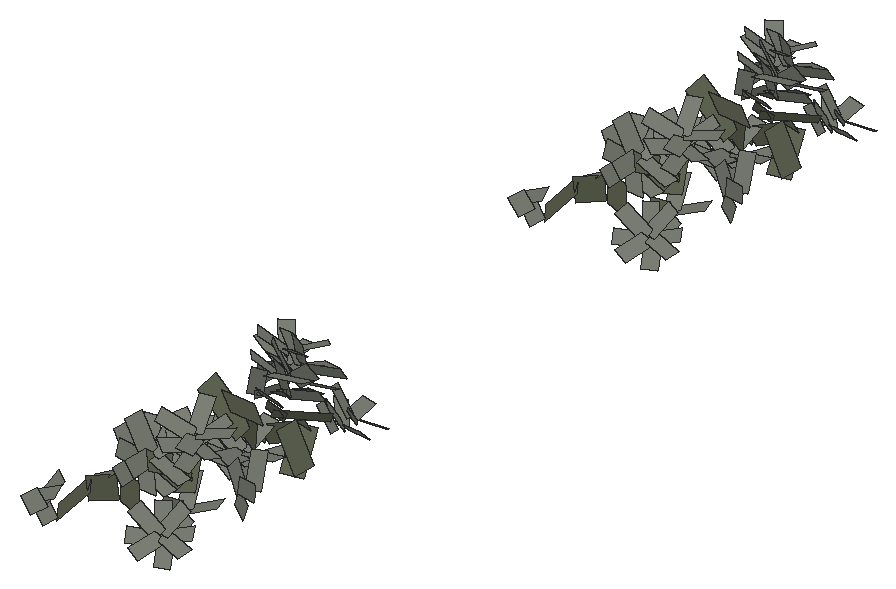
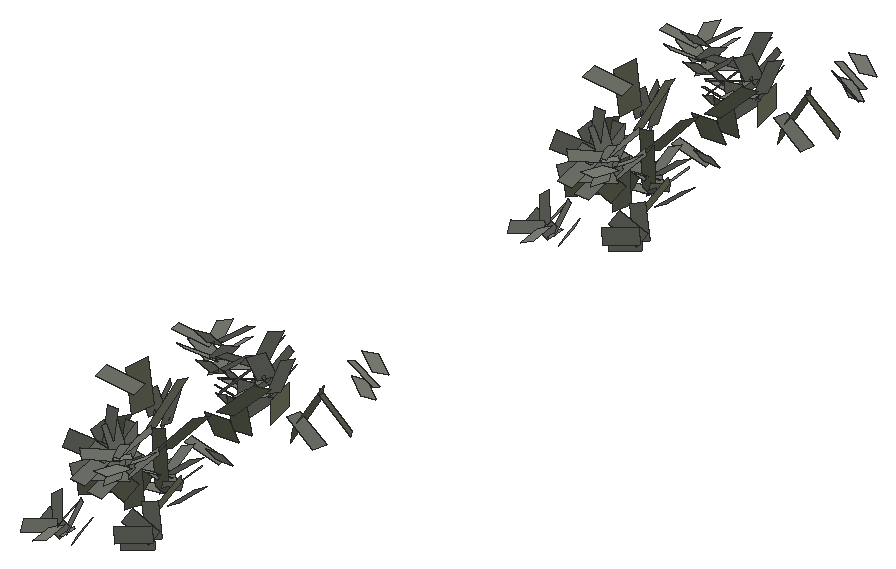
# SketchUp Ruby script. Lengths in inches.
U = 1.inch
M = Sketchup.active_model
def pt(a) = Geom::Point3d.new(a.map { |v| v * U })
def face(e, loops, mat)
  f = e.add_face(loops[0].map { |a| pt(a) })
  loops[1..].each { |l| e.add_face(l.map { |a| pt(a) }).erase! }
  f.material = f.back_material = mat if mat
  f
end
# faces: each face lists its corners as indices into pts; further lists are holes
def faces(e, pts, list, mat = nil) = list.each { |f| face(e, (f[0].is_a?(Array) ? f : [f]).map { |l| l.map { |i| pts[i] } }, mat) }
# xy, xz, yz: faces in a plane at the given z, y or x. An outline is a flat list of corners, or four numbers for a rectangle; further outlines are holes
def ring(l) = l.size == 4 ? [[l[0], l[1]], [l[2], l[1]], [l[2], l[3]], [l[0], l[3]]] : l.each_slice(2).to_a
def flat(e, list, mat, &to3) = list.each { |f| face(e, (f[0].is_a?(Array) ? f : [f]).map { |l| ring(l).map { |u, v| to3.(u, v) } }, mat) }
def xy(e, z, list, mat = nil) = flat(e, list, mat) { |x, y| [x, y, z] }
def xz(e, y, list, mat = nil) = flat(e, list, mat) { |x, z| [x, y, z] }
def yz(e, x, list, mat = nil) = flat(e, list, mat) { |y, z| [x, y, z] }
def lines(e, pts, list) = list.each { |a, b| e.add_line(pt(pts[a]), pt(pts[b])) }
# prism: a flat outline (further loops are holes) pulled along v
def prism(e, loops, v, mat = nil)
  f = face(e, loops, mat); d = Geom::Vector3d.new(v.map { |x| x * U })
  f.pushpull(f.normal.samedirection?(d) ? d.length : -d.length)
end
def box(e, o, s, mat = nil) = prism(e, [[o, [o[0] + s[0], o[1], o[2]], [o[0] + s[0], o[1] + s[1], o[2]], [o[0], o[1] + s[1], o[2]]]], [0, 0, s[2]], mat)
def at(x, y, z, deg = 0) = Geom::Transformation.translation(pt([x, y, z])) * Geom::Transformation.rotation(ORIGIN, Z_AXIS, deg.degrees)
def axes(o, x, y, z) = Geom::Transformation.new([*x, 0, *y, 0, *z, 0, *pt(o).to_a, 1])
def part(name) = M.definitions.add(name)
# library, detail: a bought-in or finely detailed component or shape, given as its bounding box
def library(name, o, s) = part(name).tap { |d| box(d.entities, o, s) }
def detail(e, o, s) = box(e.add_group.entities, o, s)
def put(e, d, t, mat = nil) = e.add_instance(d, t).tap { |i| i.material = mat if mat }
def group(e, t, mat = nil) = e.add_group.tap { |g| g.transformation = t; g.material = mat if mat }.entities
root = M.entities
M.materials.add("viburnumblaasdfas0df1w06d").color = [98, 102, 84]
M.materials.add("viburnumbladsadfasdfad0w122").color = [125, 129, 119]
c1 = part("Component\#315")
p = [[0.25,0,0],[2.05,0.01,0.35],[1.81,4.2,1.66],[0,4.19,1.3125]]
faces(c1.entities,p,[[0,1,2,3]],"viburnumbladsadfasdfad0w122")
c2 = part("viburnumblad2")
put(c2.entities,c1,axes([-19.23,-4.49,-32.18],[83.35428,0,0],[0,79.38502,0],[0,0,83.35428]))
c3 = part("Component\#314")
p = [[0.14,0,0],[2.58,0.05,0.25],[2.44,5.11,2.64],[0,5.05,2.39]]
faces(c3.entities,p,[[0,1,2,3]],"viburnumblaasdfas0df1w06d")
c4 = part("viburnumblad1\#2")
put(c4.entities,c3,axes([-37.25,6.23,19.31],[75.98784,0,0],[0,65.50676,0],[0,0,75.98784]))
put(root,c2,axes([1232.09,187.71,33.1875],[0.01038,-0.0051,-0.00415],[0.00571,0.00633,0.00604],[-0.00053,-0.00802,0.00751]))
put(root,c2,axes([1232.15,299.43,32.05],[0.00525,-0.00588,0.00776],[0.00856,0.00697,-0.00051],[-0.00462,0.00625,0.00786]))
put(root,c2,axes([1232.15,222.55,32.05],[0.00525,-0.00588,0.00776],[0.00856,0.00697,-0.00051],[-0.00462,0.00625,0.00786]))
put(root,c2,axes([1232.11,273.91,31.72],[-0.00042,-0.01207,-0.00346],[0.01224,-0.00117,0.00258],[-0.0028,-0.00328,0.0118]))
put(root,c2,axes([1232.11,197.03,31.72],[-0.00042,-0.01207,-0.00346],[0.01224,-0.00117,0.00258],[-0.0028,-0.00328,0.0118]))
put(root,c2,axes([1233.2,298.68,31.16],[-0.0027,-0.00851,0.00652],[0.00882,0.00097,0.00492],[-0.00475,0.00698,0.00714]))
put(root,c2,axes([1233.2,221.8,31.16],[-0.0027,-0.00851,0.00652],[0.00882,0.00097,0.00492],[-0.00475,0.00698,0.00714]))
put(root,c4,axes([1232.09,268.17,30.0625],[0.00746,-0.00961,-0.00443],[0.01187,0.00604,0.00656],[-0.00274,-0.0068,0.00947]))
put(root,c4,axes([1232.09,191.28,30.0625],[0.00746,-0.00961,-0.00443],[0.01187,0.00604,0.00656],[-0.00274,-0.0068,0.00947]))
put(root,c2,axes([1232.46,263.98,34.32],[0.00254,-0.00908,-0.00688],[0.01053,0.00118,0.00207],[-0.00116,-0.00732,0.00806]))
put(root,c2,axes([1232.46,187.1,34.32],[0.00254,-0.00908,-0.00688],[0.01053,0.00118,0.00207],[-0.00116,-0.00732,0.00806]))
put(root,c2,axes([1234.25,297.67,30.84],[-0.00788,-0.0064,0.00067],[0.00477,-0.00497,0.00864],[-0.00511,0.00701,0.00686]))
put(root,c2,axes([1234.25,220.79,30.84],[-0.00788,-0.0064,0.00067],[0.00477,-0.00497,0.00864],[-0.00511,0.00701,0.00686]))
put(root,c2,axes([1233.36,264.65,33.3],[-0.00572,-0.00664,-0.00612],[0.0099,-0.00571,-0.00294],[-0.00165,-0.00728,0.00803]))
put(root,c2,axes([1233.36,187.76,33.3],[-0.00572,-0.00664,-0.00612],[0.0099,-0.00571,-0.00294],[-0.00165,-0.00728,0.00803]))
put(root,c2,axes([1233.42,262.85,35.21],[-0.00636,-0.00796,-0.00575],[0.0099,-0.00571,-0.00294],[-0.00097,-0.00646,0.0087]))
put(root,c2,axes([1233.42,185.97,35.21],[-0.00636,-0.00796,-0.00575],[0.0099,-0.00571,-0.00294],[-0.00097,-0.00646,0.0087]))
put(root,c2,axes([1233.23,297.71,30.22],[0.00548,-0.00614,0.0081],[0.00771,0.00628,-0.00046],[-0.00462,0.00625,0.00786]))
put(root,c2,axes([1233.23,220.82,30.22],[0.00548,-0.00614,0.0081],[0.00771,0.00628,-0.00046],[-0.00462,0.00625,0.00786]))
put(root,c4,axes([1235.59,273.05,30.45],[-0.00612,0.00474,0.0114],[-0.00511,-0.01476,0.0034],[0.01154,-0.00234,0.00716]))
put(root,c4,axes([1235.59,196.17,30.45],[-0.00612,0.00474,0.0114],[-0.00511,-0.01476,0.0034],[0.01154,-0.00234,0.00716]))
put(root,c4,axes([1238.55,292.45,28.96],[-0.00897,0.00933,0.00213],[-0.00926,-0.01033,0.00624],[0.00527,0.00238,0.01177]))
put(root,c4,axes([1238.55,215.5625,28.96],[-0.00897,0.00933,0.00213],[-0.00926,-0.01033,0.00624],[0.00527,0.00238,0.01177]))
put(root,c2,axes([1238.65,294.53,37.13],[0.0001,0.01076,-0.00253],[-0.0107,0.00082,0.00309],[0.00316,0.0024,0.01032]))
put(root,c2,axes([1238.65,217.65,37.13],[0.0001,0.01076,-0.00253],[-0.0107,0.00082,0.00309],[0.00316,0.0024,0.01032]))
put(root,c2,axes([1238.29,271.72,35.21],[0.00119,0.01147,0.00076],[-0.00783,0.00016,0.00982],[0.00974,-0.00152,0.00779]))
put(root,c2,axes([1238.29,194.84,35.21],[0.00119,0.01147,0.00076],[-0.00783,0.00016,0.00982],[0.00974,-0.00152,0.00779]))
put(root,c2,axes([1239.2,294.49,35.76],[-0.00726,0.00696,-0.0015],[-0.00749,-0.00689,0.00431],[0.00194,0.00418,0.01005]))
put(root,c2,axes([1239.2,217.61,35.76],[-0.00726,0.00696,-0.0015],[-0.00749,-0.00689,0.00431],[0.00194,0.00418,0.01005]))
put(root,c2,axes([1238.18,295.41,38.47],[0.00778,0.00725,-0.00304],[-0.00736,0.00822,0.00077],[0.00276,0.00149,0.0106]))
put(root,c2,axes([1238.18,218.53,38.47],[0.00778,0.00725,-0.00304],[-0.00736,0.00822,0.00077],[0.00276,0.00149,0.0106]))
put(root,c2,axes([1239.56,285.86,28.45],[0.00022,0.01156,-0.00012],[-0.01157,0.00026,0.0049],[0.0049,0.00003,0.01157]))
put(root,c2,axes([1239.56,208.98,28.45],[0.00022,0.01156,-0.00012],[-0.01157,0.00026,0.0049],[0.0049,0.00003,0.01157]))
put(root,c2,axes([1239.54,295.12,38.31],[-0.00764,0.00797,-0.00053],[-0.00749,-0.00689,0.00431],[0.00278,0.00334,0.01017]))
put(root,c2,axes([1239.54,218.23,38.31],[-0.00764,0.00797,-0.00053],[-0.00749,-0.00689,0.00431],[0.00278,0.00334,0.01017]))
put(root,c2,axes([1239.13,272.51,34.5],[-0.00933,0.00053,0.0092],[-0.00115,-0.01124,-0.00052],[0.00874,-0.00131,0.00893]))
put(root,c2,axes([1239.13,195.63,34.5],[-0.00933,0.00053,0.0092],[-0.00115,-0.01124,-0.00052],[0.00874,-0.00131,0.00893]))
put(root,c2,axes([1240.31,285.66,31.36],[0.00076,0.01249,0.00112],[-0.01157,0.00026,0.0049],[0.00485,-0.00133,0.01151]))
put(root,c2,axes([1240.31,208.78,31.36],[0.00076,0.01249,0.00112],[-0.01157,0.00026,0.0049],[0.00485,-0.00133,0.01151]))
put(root,c2,axes([1237.83,295.68,37.01],[0.0109,-0.00051,-0.00178],[0.00032,0.01098,-0.00121],[0.00182,0.00115,0.01084]))
put(root,c2,axes([1237.83,218.8,37.01],[0.0109,-0.00051,-0.00178],[0.00032,0.01098,-0.00121],[0.00182,0.00115,0.01084]))
put(root,c2,axes([1239.15,286.13,30.07],[0.00907,0.00853,-0.00165],[-0.0076,0.009,0.00473],[0.00435,-0.00239,0.01154]))
put(root,c2,axes([1239.15,209.25,30.07],[0.00907,0.00853,-0.00165],[-0.0076,0.009,0.00473],[0.00435,-0.00239,0.01154]))
put(root,c4,axes([1237.12,273.84,32.35],[-0.00769,-0.00672,0.00925],[0.00492,-0.01396,-0.00605],[0.01062,-0.00006,0.00878]))
put(root,c4,axes([1237.12,196.96,32.35],[-0.00769,-0.00672,0.00925],[0.00492,-0.01396,-0.00605],[0.01062,-0.00006,0.00878]))
put(root,c2,axes([1239.95,271.76,35.57],[-0.00467,0.00901,0.00741],[-0.00631,-0.00787,0.00559],[0.00942,-0.00179,0.00811]))
put(root,c2,axes([1239.95,194.875,35.57],[-0.00467,0.00901,0.00741],[-0.00631,-0.00787,0.00559],[0.00942,-0.00179,0.00811]))
put(root,c4,axes([1240.96,285.5,33.07],[0.00029,0.0147,0.00242],[-0.01575,-0.00086,0.00709],[0.00615,-0.00232,0.01338]))
put(root,c4,axes([1240.96,208.62,33.07],[0.00029,0.0147,0.00242],[-0.01575,-0.00086,0.00709],[0.00615,-0.00232,0.01338]))
put(root,c2,axes([1238.71,271.82,36.84],[0.00797,0.00829,-0.00506],[-0.00363,0.00868,0.00851],[0.00902,-0.0039,0.00783]))
put(root,c2,axes([1238.71,194.94,36.84],[0.00797,0.00829,-0.00506],[-0.00363,0.00868,0.00851],[0.00902,-0.0039,0.00783]))
put(root,c2,axes([1239.74,295.55,36.67],[-0.0109,0.00051,0.00178],[0.00012,-0.00953,0.00349],[0.00185,0.00377,0.01023]))
put(root,c2,axes([1239.74,218.66,36.67],[-0.0109,0.00051,0.00178],[0.00012,-0.00953,0.00349],[0.00185,0.00377,0.01023]))
put(root,c2,axes([1240.84,286.07,29.54],[-0.008,0.00913,0.00324],[-0.00789,-0.00792,0.00285],[0.00448,-0.00024,0.01173]))
put(root,c2,axes([1240.84,209.19,29.54],[-0.008,0.00913,0.00324],[-0.00789,-0.00792,0.00285],[0.00448,-0.00024,0.01173]))
put(root,c2,axes([1240.97,294.75,38.1875],[0.00051,0.00894,-0.00882],[-0.0118,0.00335,0.00272],[0.00429,0.00817,0.00853]))
put(root,c2,axes([1240.97,217.87,38.1875],[0.00051,0.00894,-0.00882],[-0.0118,0.00335,0.00272],[0.00429,0.00817,0.00853]))
put(root,c2,axes([1240.06,294.05,36.89],[0.00901,0.00467,-0.00741],[-0.00789,0.00895,-0.00395],[0.00381,0.00748,0.00935]))
put(root,c2,axes([1240.06,217.17,36.89],[0.00901,0.00467,-0.00741],[-0.00789,0.00895,-0.00395],[0.00381,0.00748,0.00935]))
put(root,c2,axes([1240.3,271.16,37.375],[0.00233,0.01223,0.00166],[-0.00783,0.00016,0.00982],[0.00954,-0.00286,0.00766]))
put(root,c2,axes([1240.3,194.27,37.375],[0.00233,0.01223,0.00166],[-0.00783,0.00016,0.00982],[0.00954,-0.00286,0.00766]))
put(root,c2,axes([1241.6,293.58,36.84],[-0.00829,0.00797,-0.00506],[-0.00868,-0.00363,0.00851],[0.0039,0.00902,0.00783]))
put(root,c2,axes([1241.6,216.7,36.84],[-0.00829,0.00797,-0.00506],[-0.00868,-0.00363,0.00851],[0.0039,0.00902,0.00783]))
put(root,c4,axes([1241.5,275.36,32.19],[0.00217,0.0115,0.00524],[-0.01369,-0.00006,0.0058],[0.00451,-0.00566,0.01058]))
put(root,c4,axes([1241.5,198.47,32.19],[0.00217,0.0115,0.00524],[-0.01369,-0.00006,0.0058],[0.00451,-0.00566,0.01058]))
put(root,c2,axes([1237.95,295.79,35.54],[0.00733,-0.00766,0.00051],[0.00858,0.00809,-0.00187],[0.00089,0.00157,0.01091]))
put(root,c2,axes([1237.95,218.91,35.54],[0.00733,-0.00766,0.00051],[0.00858,0.00809,-0.00187],[0.00089,0.00157,0.01091]))
put(root,c2,axes([1239.52,277.4,28.86],[0.01126,0.00309,-0.00036],[-0.00265,0.01026,0.00493],[0.00162,-0.00467,0.01059]))
put(root,c2,axes([1239.52,200.52,28.86],[0.01126,0.00309,-0.00036],[-0.00265,0.01026,0.00493],[0.00162,-0.00467,0.01059]))
put(root,c4,axes([1239.78,276.79,30.44],[0.01321,0.00417,0.00061],[-0.00463,0.0136,0.00723],[0.00136,-0.00611,0.01237]))
put(root,c4,axes([1239.78,199.91,30.44],[0.01321,0.00417,0.00061],[-0.00463,0.0136,0.00723],[0.00136,-0.00611,0.01237]))
put(root,c2,axes([1239.34,295.62,35.38],[-0.00812,-0.00757,0.00318],[0.00703,-0.00685,0.00164],[0.0009,0.00343,0.01047]))
put(root,c2,axes([1239.34,218.74,35.38],[-0.00812,-0.00757,0.00318],[0.00703,-0.00685,0.00164],[0.0009,0.00343,0.01047]))
put(root,c4,axes([1239.15,294.31,30.8],[-0.01039,-0.00352,0.00517],[0.00601,-0.01213,0.00383],[0.0035,0.00504,0.01046]))
put(root,c4,axes([1239.15,217.42,30.8],[-0.01039,-0.00352,0.00517],[0.00601,-0.01213,0.00383],[0.0035,0.00504,0.01046]))
put(root,c2,axes([1238.43,296.74,38.12],[0.00764,-0.00797,0.00053],[0.00794,0.00749,-0.00173],[0.00089,0.00157,0.01091]))
put(root,c2,axes([1238.43,219.86,38.12],[0.00764,-0.00797,0.00053],[0.00794,0.00749,-0.00173],[0.00089,0.00157,0.01091]))
put(root,c2,axes([1238.6,273.75,35.36],[-0.00224,-0.01174,-0.0016],[0.0107,-0.00091,-0.00829],[0.00736,-0.00274,0.0098]))
put(root,c2,axes([1238.6,196.87,35.36],[-0.00224,-0.01174,-0.0016],[0.0107,-0.00091,-0.00829],[0.00736,-0.00274,0.0098]))
put(root,c2,axes([1239.78,296.44,37.95],[-0.00778,-0.00725,0.00304],[0.00781,-0.00761,0.00182],[0.0009,0.00343,0.01047]))
put(root,c2,axes([1239.78,219.5625,37.95],[-0.00778,-0.00725,0.00304],[0.00781,-0.00761,0.00182],[0.0009,0.00343,0.01047]))
put(root,c2,axes([1239.51,286.98,31.72],[0.01207,-0.00042,-0.00346],[0.00117,0.01224,0.00258],[0.00328,-0.0028,0.0118]))
put(root,c2,axes([1239.51,210.1,31.72],[0.01207,-0.00042,-0.00346],[0.00117,0.01224,0.00258],[0.00328,-0.0028,0.0118]))
put(root,c2,axes([1238.77,296.42,36.65],[-0.0001,-0.01076,0.00253],[0.0116,-0.00022,-0.00049],[0.00051,0.00252,0.01075]))
put(root,c2,axes([1238.77,219.54,36.65],[-0.0001,-0.01076,0.00253],[0.0116,-0.00022,-0.00049],[0.00051,0.00252,0.01075]))
put(root,c2,axes([1239.67,293.46,35.36],[0.01174,-0.00224,-0.0016],[0.00091,0.0107,-0.00829],[0.00274,0.00736,0.0098]))
put(root,c2,axes([1239.67,216.58,35.36],[0.01174,-0.00224,-0.0016],[0.00091,0.0107,-0.00829],[0.00274,0.00736,0.0098]))
put(root,c4,axes([1240.67,287.6,29.4],[-0.01355,0.00411,0.00465],[0.00135,-0.01078,0.01345],[0.00609,0.01091,0.00813]))
put(root,c4,axes([1240.67,210.72,29.4],[-0.01355,0.00411,0.00465],[0.00135,-0.01078,0.01345],[0.00609,0.01091,0.00813]))
put(root,c4,axes([1238.51,295.41,32.67],[-0.00272,-0.01048,0.00546],[0.01366,-0.00332,0.00044],[0.00096,0.00539,0.01082]))
put(root,c4,axes([1238.51,218.53,32.67],[-0.00272,-0.01048,0.00546],[0.01366,-0.00332,0.00044],[0.00096,0.00539,0.01082]))
put(root,c2,axes([1240.15,273.19,35.86],[-0.00797,-0.00829,0.00506],[0.00596,-0.00975,-0.0066],[0.00788,-0.0017,0.00963]))
put(root,c2,axes([1240.15,196.3125,35.86],[-0.00797,-0.00829,0.00506],[0.00596,-0.00975,-0.0066],[0.00788,-0.0017,0.00963]))
put(root,c2,axes([1241.62,286.52,31.08],[-0.01207,0.00042,0.00346],[-0.00034,-0.01255,0.00035],[0.00347,0.00024,0.01207]))
put(root,c2,axes([1241.62,209.64,31.08],[-0.01207,0.00042,0.00346],[-0.00034,-0.01255,0.00035],[0.00347,0.00024,0.01207]))
put(root,c2,axes([1241.39,271.99,36.58],[-0.00894,0.00051,0.00882],[-0.00128,-0.01248,-0.00058],[0.00874,-0.00131,0.00893]))
put(root,c2,axes([1241.39,195.11,36.58],[-0.00894,0.00051,0.00882],[-0.00128,-0.01248,-0.00058],[0.00874,-0.00131,0.00893]))
put(root,c2,axes([1241.7,293.15,35.21],[-0.01147,0.00119,0.00076],[-0.00016,-0.00783,0.00982],[0.00152,0.00974,0.00779]))
put(root,c2,axes([1241.7,216.27,35.21],[-0.01147,0.00119,0.00076],[-0.00016,-0.00783,0.00982],[0.00152,0.00974,0.00779]))
put(root,c2,axes([1240.13,295.85,37.4],[0.01223,-0.00233,-0.00166],[0.00085,0.00991,-0.00768],[0.00274,0.00736,0.0098]))
put(root,c2,axes([1240.13,218.96,37.4],[0.01223,-0.00233,-0.00166],[0.00085,0.00991,-0.00768],[0.00274,0.00736,0.0098]))
put(root,c2,axes([1239.18,273.36,36.89],[0.00467,-0.00901,-0.00741],[0.00895,0.00789,-0.00395],[0.00748,-0.00381,0.00935]))
put(root,c2,axes([1239.18,196.48,36.89],[0.00467,-0.00901,-0.00741],[0.00895,0.00789,-0.00395],[0.00748,-0.00381,0.00935]))
put(root,c2,axes([1242.55,298.26,29.06],[-0.00329,0.00963,-0.00365],[-0.00749,-0.00039,0.00532],[0.00532,0.00466,0.00661]))
put(root,c2,axes([1242.55,221.375,29.06],[-0.00329,0.00963,-0.00365],[-0.00749,-0.00039,0.00532],[0.00532,0.00466,0.00661]))
put(root,c2,axes([1239.89,272.46,38.1875],[0.00894,-0.00051,-0.00882],[0.00335,0.0118,0.00272],[0.00817,-0.00429,0.00853]))
put(root,c2,axes([1239.89,195.57,38.1875],[0.00894,-0.00051,-0.00882],[0.00335,0.0118,0.00272],[0.00817,-0.00429,0.00853]))
put(root,c2,axes([1242.27,295.16,37.375],[-0.01223,0.00233,0.00166],[-0.00016,-0.00783,0.00982],[0.00286,0.00954,0.00766]))
put(root,c2,axes([1242.27,218.28,37.375],[-0.01223,0.00233,0.00166],[-0.00016,-0.00783,0.00982],[0.00286,0.00954,0.00766]))
put(root,c2,axes([1239.48,287.71,30.15],[0.008,-0.00913,-0.00324],[0.00942,0.00831,-0.00017],[0.00227,-0.00232,0.01214]))
put(root,c2,axes([1239.48,210.83,30.15],[0.008,-0.00913,-0.00324],[0.00942,0.00831,-0.00017],[0.00227,-0.00232,0.01214]))
put(root,c2,axes([1243.24,274.57,36.85],[-0.00295,0.01122,0.00376],[-0.00948,-0.00348,0.00294],[0.00419,-0.00245,0.01063]))
put(root,c2,axes([1243.24,197.68,36.85],[-0.00295,0.01122,0.00376],[-0.00948,-0.00348,0.00294],[0.00419,-0.00245,0.01063]))
put(root,c4,axes([1243.07,275.45,33.98],[-0.00789,0.00746,0.00681],[-0.00938,-0.01142,0.00165],[0.00606,-0.00342,0.01077]))
put(root,c4,axes([1243.07,198.57,33.98],[-0.00789,0.00746,0.00681],[-0.00938,-0.01142,0.00165],[0.00606,-0.00342,0.01077]))
put(root,c2,axes([1240.82,287.54,29.72],[-0.00907,-0.00853,0.00165],[0.00877,-0.00968,-0.00184],[0.0024,-0.00017,0.01233]))
put(root,c2,axes([1240.82,210.66,29.72],[-0.00907,-0.00853,0.00165],[0.00877,-0.00968,-0.00184],[0.0024,-0.00017,0.01233]))
put(root,c2,axes([1242.7,298.86,30.05],[0.00407,0.00723,-0.00605],[-0.00729,0.00582,0.00182],[0.00528,0.00383,0.00709]))
put(root,c2,axes([1242.7,221.98,30.05],[0.00407,0.00723,-0.00605],[-0.00729,0.00582,0.00182],[0.00528,0.00383,0.00709]))
put(root,c4,axes([1242.93,286.52,35.17],[-0.01118,0.00552,0.00587],[-0.00491,-0.01458,0.00435],[0.00686,0.00124,0.01189]))
put(root,c4,axes([1242.93,209.63,35.17],[-0.01118,0.00552,0.00587],[-0.00491,-0.01458,0.00435],[0.00686,0.00124,0.01189]))
put(root,c2,axes([1243.16,274.22,38.23],[0.00575,0.0101,0.00117],[-0.00857,0.00432,0.00479],[0.00404,-0.00351,0.01039]))
put(root,c2,axes([1243.16,197.34,38.23],[0.00575,0.0101,0.00117],[-0.00857,0.00432,0.00479],[0.00404,-0.00351,0.01039]))
put(root,c2,axes([1241.67,294.8125,35.57],[-0.00901,-0.00467,0.00741],[0.00787,-0.00631,0.00559],[0.00179,0.00942,0.00811]))
put(root,c2,axes([1241.67,217.93,35.57],[-0.00901,-0.00467,0.00741],[0.00787,-0.00631,0.00559],[0.00179,0.00942,0.00811]))
put(root,c2,axes([1243.78,299.28,30.83],[-0.00315,0.00923,-0.0035],[-0.00832,-0.00043,0.00591],[0.00532,0.00466,0.00661]))
put(root,c2,axes([1243.78,222.4,30.83],[-0.00315,0.00923,-0.0035],[-0.00832,-0.00043,0.00591],[0.00532,0.00466,0.00661]))
put(root,c2,axes([1244.16,273.76,39.47],[-0.00283,0.01075,0.0036],[-0.01053,-0.00387,0.00326],[0.00419,-0.00245,0.01063]))
put(root,c2,axes([1244.16,196.875,39.47],[-0.00283,0.01075,0.0036],[-0.01053,-0.00387,0.00326],[0.00419,-0.00245,0.01063]))
put(root,c4,axes([1239.59,291.99,32.35],[0.00672,-0.00769,0.00925],[0.01396,0.00492,-0.00605],[0.00006,0.01062,0.00878]))
put(root,c4,axes([1239.59,215.1,32.35],[0.00672,-0.00769,0.00925],[0.01396,0.00492,-0.00605],[0.00006,0.01062,0.00878]))
put(root,c2,axes([1240.23,295.01,35.86],[0.00829,-0.00797,0.00506],[0.00975,0.00596,-0.0066],[0.0017,0.00788,0.00963]))
put(root,c2,axes([1240.23,218.13,35.86],[0.00829,-0.00797,0.00506],[0.00975,0.00596,-0.0066],[0.0017,0.00788,0.00963]))
put(root,c2,axes([1240.48,278.5,29.09],[0.00283,-0.01075,-0.0036],[0.01134,0.00265,0.001],[-0.0001,-0.00373,0.01107]))
put(root,c2,axes([1240.48,201.62,29.09],[0.00283,-0.01075,-0.0036],[0.01134,0.00265,0.001],[-0.0001,-0.00373,0.01107]))
put(root,c2,axes([1243.82,269.34,29.19],[0.00369,0.00856,0.00471],[-0.00994,0.00059,0.00626],[0.00445,-0.00629,0.00669]))
put(root,c2,axes([1243.82,192.46,29.19],[0.00369,0.00856,0.00471],[-0.00994,0.00059,0.00626],[0.00445,-0.00629,0.00669]))
put(root,c2,axes([1240.98,273.29,37.4],[-0.00233,-0.01223,-0.00166],[0.00991,-0.00085,-0.00768],[0.00736,-0.00274,0.0098]))
put(root,c2,axes([1240.98,196.41,37.4],[-0.00233,-0.01223,-0.00166],[0.00991,-0.00085,-0.00768],[0.00736,-0.00274,0.0098]))
put(root,c2,axes([1242.3,275.22,37.36],[0.00971,0.00365,-0.00281],[-0.00246,0.01032,0.00491],[0.00437,-0.00379,0.01015]))
put(root,c2,axes([1242.3,198.34,37.36],[0.00971,0.00365,-0.00281],[-0.00246,0.01032,0.00491],[0.00437,-0.00379,0.01015]))
put(root,c2,axes([1243.72,299.07,29.43],[-0.00853,0.00582,0.00111],[-0.0037,-0.00695,0.00724],[0.00473,0.00542,0.00649]))
put(root,c2,axes([1243.72,222.18,29.43],[-0.00853,0.00582,0.00111],[-0.0037,-0.00695,0.00724],[0.00473,0.00542,0.00649]))
put(root,c2,axes([1240.91,294,34.5],[-0.00053,-0.00933,0.0092],[0.01124,-0.00115,-0.00052],[0.00131,0.00874,0.00893]))
put(root,c2,axes([1240.91,217.12,34.5],[-0.00053,-0.00933,0.0092],[0.01124,-0.00115,-0.00052],[0.00131,0.00874,0.00893]))
put(root,c2,axes([1240.82,287.84,31.45],[-0.00076,-0.01249,-0.00112],[0.01239,-0.00058,-0.00197],[0.0019,-0.00123,0.01236]))
put(root,c2,axes([1240.82,210.96,31.45],[-0.00076,-0.01249,-0.00112],[0.01239,-0.00058,-0.00197],[0.0019,-0.00123,0.01236]))
put(root,c4,axes([1240.375,290.45,30.45],[-0.00474,-0.00612,0.0114],[0.01476,-0.00511,0.0034],[0.00234,0.01154,0.00716]))
put(root,c4,axes([1240.375,213.57,30.45],[-0.00474,-0.00612,0.0114],[0.01476,-0.00511,0.0034],[0.00234,0.01154,0.00716]))
put(root,c4,axes([1242.37,271.41,28],[0.0118,0.00221,-0.00034],[-0.00169,0.00933,0.00984],[0.00149,-0.00861,0.00716]))
put(root,c4,axes([1242.37,194.53,28],[0.0118,0.00221,-0.00034],[-0.00169,0.00933,0.00984],[0.00149,-0.00861,0.00716]))
put(root,c2,axes([1244.43,274.73,38.05],[-0.00975,0.0051,0.00392],[-0.00563,-0.0109,0.00018],[0.00356,-0.00165,0.01101]))
put(root,c2,axes([1244.43,197.85,38.05],[-0.00975,0.0051,0.00392],[-0.00563,-0.0109,0.00018],[0.00356,-0.00165,0.01101]))
put(root,c2,axes([1242.8,300.16,30.84],[0.00891,0.00099,-0.00506],[-0.00261,0.00972,-0.00258],[0.00462,0.00341,0.00766]))
put(root,c2,axes([1242.8,223.28,30.84],[0.00891,0.00099,-0.00506],[-0.00261,0.00972,-0.00258],[0.00462,0.00341,0.00766]))
put(root,c2,axes([1244.74,268.56,29.87],[-0.00413,0.00723,0.00696],[-0.00909,-0.00609,0.00092],[0.00444,-0.00548,0.00729]))
put(root,c2,axes([1244.74,191.68,29.87],[-0.00413,0.00723,0.00696],[-0.00909,-0.00609,0.00092],[0.00444,-0.00548,0.00729]))
put(root,c2,axes([1244.35,267.64,31.03],[0.00385,0.00891,0.00491],[-0.00921,0.00054,0.0058],[0.00445,-0.00629,0.00669]))
put(root,c2,axes([1244.35,190.75,31.03],[0.00385,0.00891,0.00491],[-0.00921,0.00054,0.0058],[0.00445,-0.00629,0.00669]))
put(root,c2,axes([1241.43,296.26,36.58],[-0.00051,-0.00894,0.00882],[0.01248,-0.00128,-0.00058],[0.00131,0.00874,0.00893]))
put(root,c2,axes([1241.43,219.375,36.58],[-0.00051,-0.00894,0.00882],[0.01248,-0.00128,-0.00058],[0.00131,0.00874,0.00893]))
put(root,c2,axes([1243.07,274.61,39.99],[0.01096,0.00354,-0.00194],[-0.00246,0.01032,0.00491],[0.0032,-0.00419,0.01042]))
put(root,c2,axes([1243.07,197.73,39.99],[0.01096,0.00354,-0.00194],[-0.00246,0.01032,0.00491],[0.0032,-0.00419,0.01042]))
put(root,c2,axes([1243.68,268.81,30.46],[0.00956,0.00538,-0.00002],[-0.00388,0.00674,0.0082],[0.00377,-0.00701,0.00644]))
put(root,c2,axes([1243.68,191.92,30.46],[0.00956,0.00538,-0.00002],[-0.00388,0.00674,0.0082],[0.00377,-0.00701,0.00644]))
put(root,c2,axes([1244.07,275.8,36.92],[-0.01053,-0.0034,0.00186],[0.00341,-0.01191,-0.00242],[0.00251,-0.00157,0.0113]))
put(root,c2,axes([1244.07,198.92,36.92],[-0.01053,-0.0034,0.00186],[0.00341,-0.01191,-0.00242],[0.00251,-0.00157,0.0113]))
put(root,c2,axes([1242.77,275.73,38.77],[0.00975,-0.0051,-0.00392],[0.00612,0.00977,0.00252],[0.00215,-0.00412,0.01072]))
put(root,c2,axes([1242.77,198.85,38.77],[0.00975,-0.0051,-0.00392],[0.00612,0.00977,0.00252],[0.00215,-0.00412,0.01072]))
put(root,c2,axes([1245.63,268.15,30.88],[-0.00968,0.00131,0.00494],[-0.00342,-0.0096,-0.00398],[0.00374,-0.00505,0.00789]))
put(root,c2,axes([1245.63,191.27,30.88],[-0.00968,0.00131,0.00494],[-0.00342,-0.0096,-0.00398],[0.00374,-0.00505,0.00789]))
put(root,c2,axes([1244.47,300.05,30.05],[-0.00891,-0.00099,0.00506],[0.00365,-0.0086,0.00436],[0.00385,0.00566,0.0068]))
put(root,c2,axes([1244.47,223.17,30.05],[-0.00891,-0.00099,0.00506],[0.00365,-0.0086,0.00436],[0.00385,0.00566,0.0068]))
put(root,c4,axes([1243.3,287.92,37.29],[-0.01061,-0.00623,0.0062],[0.00831,-0.01365,0.0005],[0.0051,0.00356,0.0123]))
put(root,c4,axes([1243.3,211.03,37.29],[-0.01061,-0.00623,0.0062],[0.00831,-0.01365,0.0005],[0.0051,0.00356,0.0123]))
put(root,c2,axes([1243.46,300.125,29.01],[-0.00407,-0.00723,0.00605],[0.00898,-0.00522,-0.00021],[0.0032,0.00525,0.00736]))
put(root,c2,axes([1243.46,223.24,29.01],[-0.00407,-0.00723,0.00605],[0.00898,-0.00522,-0.00021],[0.0032,0.00525,0.00736]))
put(root,c2,axes([1243.41,270.29,30.09],[0.01011,-0.00136,-0.00516],[0.0038,0.00729,0.00519],[0.0028,-0.00722,0.00669]))
put(root,c2,axes([1243.41,193.41,30.09],[0.01011,-0.00136,-0.00516],[0.0038,0.00729,0.00519],[0.0028,-0.00722,0.00669]))
put(root,c2,axes([1245.08,274.91,39.53],[-0.01096,-0.00354,0.00194],[0.00316,-0.01102,-0.00224],[0.00251,-0.00157,0.0113]))
put(root,c2,axes([1245.08,198.02,39.53],[-0.01096,-0.00354,0.00194],[0.00316,-0.01102,-0.00224],[0.00251,-0.00157,0.0113]))
put(root,c2,axes([1243.49,300.93,30.06],[0.00315,-0.00923,0.0035],[0.00936,0.00154,-0.00413],[0.00315,0.00442,0.00785]))
put(root,c2,axes([1243.49,224.05,30.06],[0.00315,-0.00923,0.0035],[0.00936,0.00154,-0.00413],[0.00315,0.00442,0.00785]))
put(root,c2,axes([1243.16,288.67,40.56],[-0.00026,-0.01204,0.00058],[0.0134,-0.00039,-0.00212],[0.00198,0.00055,0.01239]))
put(root,c2,axes([1243.16,211.79,40.56],[-0.00026,-0.01204,0.00058],[0.0134,-0.00039,-0.00212],[0.00198,0.00055,0.01239]))
put(root,c2,axes([1244.04,268.65,31.9],[0.00968,-0.00131,-0.00494],[0.00422,0.00809,0.00577],[0.0028,-0.00722,0.00669]))
put(root,c2,axes([1244.04,191.77,31.9],[0.00968,-0.00131,-0.00494],[0.00422,0.00809,0.00577],[0.0028,-0.00722,0.00669]))
put(root,c2,axes([1244.22,275.97,38.46],[-0.00575,-0.0101,-0.00117],[0.01003,-0.00542,-0.00255],[0.00167,-0.00226,0.01134]))
put(root,c2,axes([1244.22,199.09,38.46],[-0.00575,-0.0101,-0.00117],[0.01003,-0.00542,-0.00255],[0.00167,-0.00226,0.01134]))
put(root,c4,axes([1245.26,286.96,30.0625],[0.00961,0.00746,-0.00443],[-0.00604,0.01187,0.00656],[0.0068,-0.00274,0.00947]))
put(root,c4,axes([1245.26,210.07,30.0625],[0.00961,0.00746,-0.00443],[-0.00604,0.01187,0.00656],[0.0068,-0.00274,0.00947]))
put(root,c2,axes([1245.42,269.67,30.39],[-0.00956,-0.00538,0.00002],[0.00454,-0.00801,-0.00608],[0.00277,-0.00525,0.00814]))
put(root,c2,axes([1245.42,192.79,30.39],[-0.00956,-0.00538,0.00002],[0.00454,-0.00801,-0.00608],[0.00277,-0.00525,0.00814]))
put(root,c2,axes([1244.04,269.87,31.07],[0.00413,-0.00723,-0.00696],[0.00908,0.00421,0.0008],[0.0021,-0.00679,0.00729]))
put(root,c2,axes([1244.04,192.99,31.07],[0.00413,-0.00723,-0.00696],[0.00908,0.00421,0.0008],[0.0021,-0.00679,0.00729]))
put(root,c2,axes([1243.99,275.76,40.05],[0.00283,-0.01075,-0.0036],[0.01123,0.00316,-0.00059],[0.00152,-0.00332,0.0111]))
put(root,c2,axes([1243.99,198.875,40.05],[0.00283,-0.01075,-0.0036],[0.01123,0.00316,-0.00059],[0.00152,-0.00332,0.0111]))
put(root,c2,axes([1246.93,278.4375,31.54],[-0.0023,0.01045,0.001],[-0.00575,-0.00222,0.00993],[0.00986,0.00159,0.00606]))
put(root,c2,axes([1246.93,201.55,31.54],[-0.0023,0.01045,0.001],[-0.00575,-0.00222,0.00993],[0.00986,0.00159,0.00606]))
put(root,c2,axes([1245.32,269.17,31.75],[-0.00385,-0.00891,-0.00491],[0.01001,-0.00205,-0.00401],[0.00209,-0.00597,0.00789]))
put(root,c2,axes([1245.32,192.28,31.75],[-0.00385,-0.00891,-0.00491],[0.01001,-0.00205,-0.00401],[0.00209,-0.00597,0.00789]))
put(root,c4,axes([1247.43,286.55,30.82],[0.00184,0.01273,0.00122],[-0.0105,0.00029,0.01027],[0.00896,-0.0024,0.00784]))
put(root,c4,axes([1247.43,209.67,30.82],[0.00184,0.01273,0.00122],[-0.0105,0.00029,0.01027],[0.00896,-0.0024,0.00784]))
put(root,c2,axes([1247.46,278.65,33.01],[0.0039,0.00969,-0.00523],[-0.00478,0.00655,0.00858],[0.00995,-0.00072,0.00609]))
put(root,c2,axes([1247.46,201.77,33.01],[0.0039,0.00969,-0.00523],[-0.00478,0.00655,0.00858],[0.00995,-0.00072,0.00609]))
put(root,c2,axes([1247.35,279.39,30.83],[-0.00724,-0.00234,0.00954],[0.00229,-0.01023,-0.00078],[0.00905,0.00148,0.00724]))
put(root,c2,axes([1247.35,202.5,30.83],[-0.00724,-0.00234,0.00954],[0.00229,-0.01023,-0.00078],[0.00905,0.00148,0.00724]))
put(root,c2,axes([1248.41,278.97,31.7],[-0.00591,0.00652,0.00769],[-0.00251,-0.00882,0.00556],[0.0097,0.00126,0.00639]))
put(root,c2,axes([1248.41,202.08,31.7],[-0.00591,0.00652,0.00769],[-0.00251,-0.00882,0.00556],[0.0097,0.00126,0.00639]))
